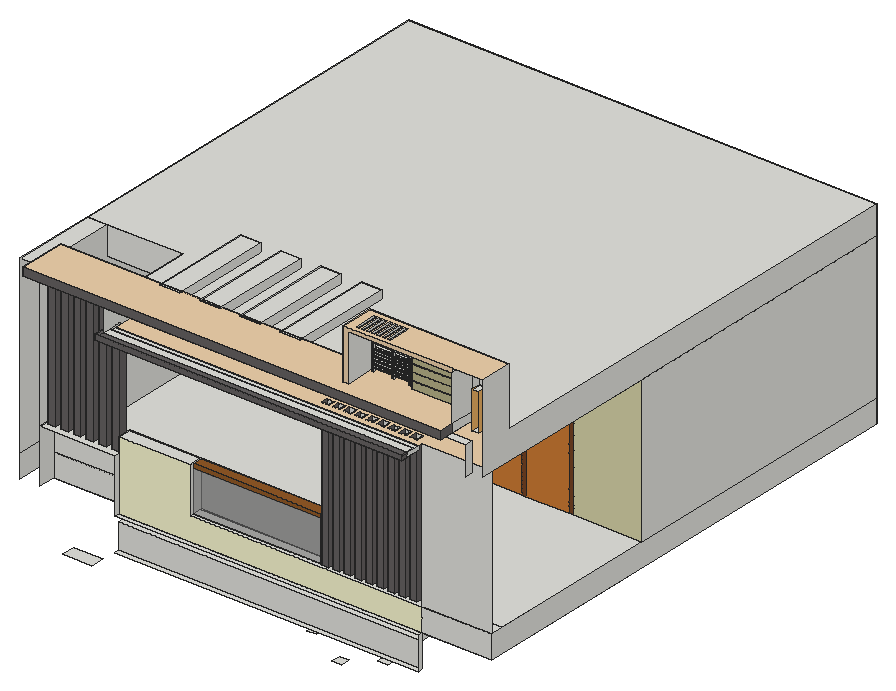
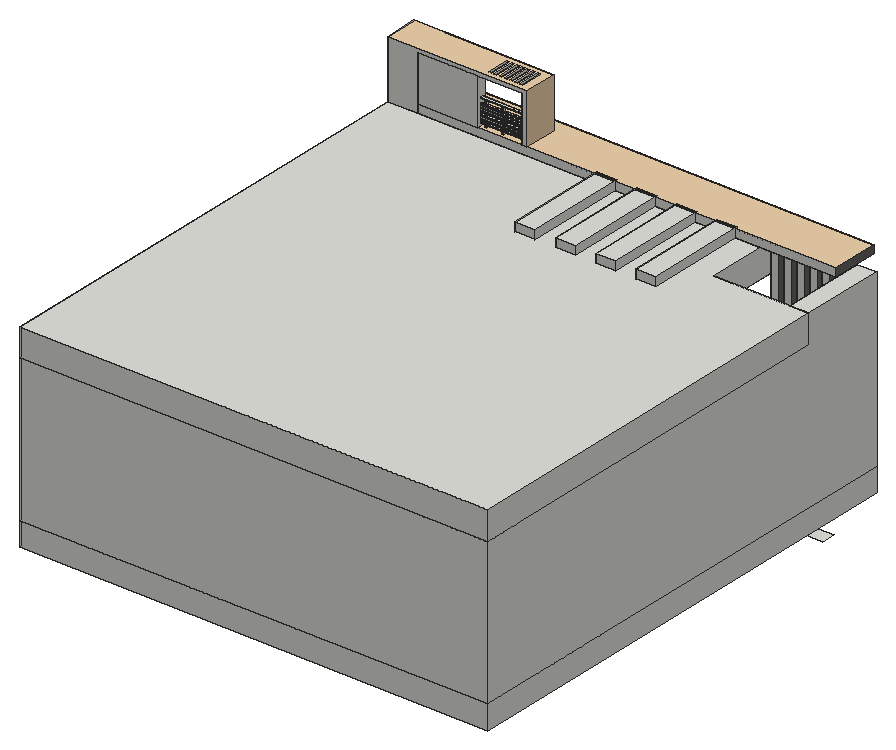
# SketchUp Ruby script. Lengths in inches.
U = 1.inch
M = Sketchup.active_model
def pt(a) = Geom::Point3d.new(a.map { |v| v * U })
def face(e, loops, mat)
  f = e.add_face(loops[0].map { |a| pt(a) })
  loops[1..].each { |l| e.add_face(l.map { |a| pt(a) }).erase! }
  f.material = f.back_material = mat if mat
  f
end
# faces: each face lists its corners as indices into pts; further lists are holes
def faces(e, pts, list, mat = nil) = list.each { |f| face(e, (f[0].is_a?(Array) ? f : [f]).map { |l| l.map { |i| pts[i] } }, mat) }
# xy, xz, yz: faces in a plane at the given z, y or x. An outline is a flat list of corners, or four numbers for a rectangle; further outlines are holes
def ring(l) = l.size == 4 ? [[l[0], l[1]], [l[2], l[1]], [l[2], l[3]], [l[0], l[3]]] : l.each_slice(2).to_a
def flat(e, list, mat, &to3) = list.each { |f| face(e, (f[0].is_a?(Array) ? f : [f]).map { |l| ring(l).map { |u, v| to3.(u, v) } }, mat) }
def xy(e, z, list, mat = nil) = flat(e, list, mat) { |x, y| [x, y, z] }
def xz(e, y, list, mat = nil) = flat(e, list, mat) { |x, z| [x, y, z] }
def yz(e, x, list, mat = nil) = flat(e, list, mat) { |y, z| [x, y, z] }
def lines(e, pts, list) = list.each { |a, b| e.add_line(pt(pts[a]), pt(pts[b])) }
# prism: a flat outline (further loops are holes) pulled along v
def prism(e, loops, v, mat = nil)
  f = face(e, loops, mat); d = Geom::Vector3d.new(v.map { |x| x * U })
  f.pushpull(f.normal.samedirection?(d) ? d.length : -d.length)
end
def box(e, o, s, mat = nil) = prism(e, [[o, [o[0] + s[0], o[1], o[2]], [o[0] + s[0], o[1] + s[1], o[2]], [o[0], o[1] + s[1], o[2]]]], [0, 0, s[2]], mat)
def at(x, y, z, deg = 0) = Geom::Transformation.translation(pt([x, y, z])) * Geom::Transformation.rotation(ORIGIN, Z_AXIS, deg.degrees)
def axes(o, x, y, z) = Geom::Transformation.new([*x, 0, *y, 0, *z, 0, *pt(o).to_a, 1])
def part(name) = M.definitions.add(name)
# library, detail: a bought-in or finely detailed component or shape, given as its bounding box
def library(name, o, s) = part(name).tap { |d| box(d.entities, o, s) }
def detail(e, o, s) = box(e.add_group.entities, o, s)
def put(e, d, t, mat = nil) = e.add_instance(d, t).tap { |i| i.material = mat if mat }
def group(e, t, mat = nil) = e.add_group.tap { |g| g.transformation = t; g.material = mat if mat }.entities
root = M.entities
M.materials.add("Generic\#1").color = [235, 176, 99]
M.materials.add("Generic\#2").color = [102, 98, 98]
M.materials.add("Generic\#3").color = [183, 179, 137]
M.materials.add("Generic\#4").color = [217, 213, 170]
M.materials.add("Generic\#6").color = [239, 209, 171]
M.materials.add("Generic\#7").color = [249, 247, 208]
M.materials.add("[Translucent Glass Gray]").color = [128, 128, 128]
M.materials["[Translucent Glass Gray]"].alpha = 0.5
M.materials.add("[Wood Bamboo]").color = [206, 124, 53]
M.materials.add("[Wood Floor Parquet]").color = [145, 89, 39]
M.materials.add("[Wood Veneer 01]").color = [119, 69, 36]
c1 = library("Group14",[-64.97,9.24,0.31],[138.52,9.93,292.57])
c2 = library("Group16",[86.37,-10.76,76.46],[21.79,14.87,35.97])
c3 = library("Group22",[48.82,-10.91,0.23],[97.72,18.57,293.12])
c4 = library("Group24",[44.03,2.01,0.26],[103.73,11,292.35])
c5 = library("Group27",[-106.21,-10.76,76.46],[21.8,14.87,35.97])
c6 = library("Group35",[-145.81,2.01,0.26],[103.73,11,292.35])
c7 = library("Group33",[-144.59,-10.91,0.23],[97.72,18.57,293.12])
c8 = part("rem (1)")
g1 = group(c8.entities,at(-145.81,-10.91,0.23))
put(g1,c1,at(145.81,10.91,-0.23))
put(g1,c2,at(145.81,10.91,-0.23))
put(g1,c3,at(145.81,10.91,-0.23))
put(g1,c4,at(145.81,10.91,-0.23))
put(g1,c5,at(145.81,10.91,-0.23))
put(g1,c6,at(145.81,10.91,-0.23))
put(g1,c7,at(145.81,10.91,-0.23))
xy(root,245.22,[[294.23,85.3125,304.04,94.5625]])
xy(root,258.96,[[42.04,67.875,71.06,81.625]])
xy(root,261.43,[[339.93,85.3125,349.75,94.5625]])
xy(root,263.68,[[269.72,85.3125,279.54,94.5625]])
xy(root,276.62,[[315.33,85.3125,325.14,94.5625]])
xy(root,277.23,[[366.08,85.3125,375.89,94.5625]])
xy(root,278.625,[[93.91,67.875,394.04,72.375]])
xy(root,286.8125,[[62.44,244.125,235.88,281.25]])
xy(root,304.1875,[[93.91,72.375,394.04,85.3125]])
xy(root,311.1875,[[93.91,67.875,394.04,72.375],[93.91,72.375,394.04,85.3125],[394.04,72.375,462.8125,85.3125]])
xy(root,311.1875,[[19.1875,85.3125,19.1875,244.125,462.8125,244.125,462.8125,94.5625,258.25,94.5625,258.25,85.3125]],"Generic\#6")
xy(root,334.375,[[[164.77,72.375,164.77,75.34,291.73,75.34,291.73,85.3125,394.04,85.3125,394.04,82.29,393.29,82.29,393.29,75.21,394.04,75.21,394.04,72.375],[291.98,75.21,299.23,82.29],[302.92,75.21,310.17,82.29],[313.86,75.21,321.11,82.29],[324.79,75.21,332.04,82.29],[335.73,75.21,342.98,82.29],[346.67,75.21,353.92,82.29],[357.92,75.21,364.86,82.29],[368.86,75.21,375.79,82.29],[379.79,75.21,386.73,82.29]],[394.04,72.375,394.04,75.21,397.67,75.21,397.67,82.29,394.04,82.29,394.04,85.3125,462.8125,85.3125,462.8125,72.375],[291.98,75.21,299.23,82.29],[302.92,75.21,310.17,82.29],[313.86,75.21,321.11,82.29],
  [324.79,75.21,332.04,82.29],[335.73,75.21,342.98,82.29],[346.67,75.21,353.92,82.29],[357.92,75.21,364.86,82.29],[368.86,75.21,375.79,82.29],
  [379.79,75.21,386.73,82.29],[393.29,75.21,394.04,82.29],[394.04,75.21,397.67,82.29],[164.77,75.34,291.73,85.3125],[19.1875,85.3125,19.1875,244.125,62.44,244.125,62.44,281.25,235.88,281.25,235.88,244.125,270.7,244.125,270.7,257.625,462.8125,257.625,462.8125,85.3125]])
xy(root,364.3125,[[[19.1875,67.875,93.91,85.3125],[21.625,74.83,29.4375,82.21],[34.25,74.83,42.0625,82.21],[46.875,74.83,54.6875,82.21],[59.5,74.83,67.3125,82.21],[72.125,74.83,79.9375,82.21],[84.75,74.83,92.5625,82.21]]])
xy(root,375.4375,[[164.77,75.34,291.73,85.3125]])
xy(root,379.375,[[93.91,72.375,164.77,85.3125]])
xy(root,379.375,[[164.77,75.34,291.73,85.3125]],"[Wood Floor Parquet]")
xy(root,454,[[62.44,244.125,235.88,281.25]])
xy(root,474.875,[[90.47,47.0625,90.47,74.83,93.91,74.83,93.91,67.875,394.04,67.875,394.04,47.0625]])
xy(root,478.375,[[93.91,60.6875,394.04,67.875],[0,151.0625,0,547.875,462.8125,547.875,462.8125,257.625,270.7,257.625,270.7,244.125,19.1875,244.125,19.1875,151.0625]])
xy(root,478.375,[[[93.91,67.875,93.91,151.0625,19.1875,151.0625,19.1875,244.125,270.7,244.125,270.7,257.625,462.8125,257.625,462.8125,72.375,394.04,72.375,394.04,67.875],[119.28,91.33,139.09,191.7],[158.97,91.33,178.78,191.7],[198.65,91.33,218.47,191.7],[238.34,91.33,258.15,191.7],[346.67,75.21,353.92,82.29],[335.73,75.21,342.98,82.29],[324.79,75.21,332.04,82.29],[313.86,75.21,321.11,82.29],[302.92,75.21,310.17,82.29],[291.98,75.21,299.23,82.29],[379.79,75.21,386.73,82.29],[368.86,75.21,375.79,82.29],[357.92,75.21,364.86,82.29]]],"Generic\#6")
xy(root,480.125,[[93.91,53.25,394.04,60.6875]])
xy(root,480.125,[[90.47,47.0625,93.91,74.83],[93.91,47.0625,394.04,53.25]],"Generic\#2")
xy(root,506.6875,[[[19.1875,47.0625,93.91,93.625],[21.625,74.83,29.4375,82.21],[34.25,74.83,42.0625,82.21],[46.875,74.83,54.6875,82.21],[59.5,74.83,67.3125,82.21],[72.125,74.83,79.9375,82.21],[84.75,74.83,92.5625,82.21]],[93.91,47.0625,432.56,53.25],[93.91,53.25,432.56,93.625],[432.56,53.25,452.8125,60.6875],[0,67.875,19.1875,151.0625],
  [93.91,93.625,462.8125,93.625,462.8125,547.875,0,547.875,0,151.0625,93.91,151.0625]])
xy(root,514.6875,[[374,85,432.56,93.625],[332.03,87.87,333.97,89.37],[351.41,87.87,353.35,89.37],[368.3,88.125,370.24,89.3125],[119.28,91.33,139.09,93.625],
  [158.97,91.33,178.78,93.625],[198.65,91.33,218.47,93.625],[238.34,91.33,258.15,93.625],[119.28,93.625,139.09,191.7],[158.97,93.625,178.78,191.7],
  [198.65,93.625,218.47,191.7],[238.34,93.625,258.15,191.7]])
xy(root,514.6875,[[[19.1875,47.0625,432.56,47.0625,432.56,85,374,85,374,93.625,330.5,93.625,330.5,60.6875,325.13,60.6875,325.13,93.625,258.15,93.625,258.15,91.33,238.34,91.33,238.34,93.625,218.47,93.625,218.47,91.33,198.65,91.33,198.65,93.625,178.78,93.625,178.78,91.33,158.97,91.33,158.97,93.625,139.09,93.625,139.09,91.33,119.28,91.33,119.28,93.625,19.1875,93.625],[351.41,87.87,353.35,89.37],[332.03,87.87,333.97,89.37],[368.3,88.125,370.24,89.3125]]],"Generic\#6")
xy(root,515.875,[[452.8125,60.6875,459.25,69.875]])
xy(root,517.37,[[330.5,87.99,374,90.49]])
xy(root,518.43,[[330.5,87.99,374,90.49]])
xy(root,519.93,[[330.5,87.99,374,90.49]])
xy(root,520.99,[[330.5,87.99,374,90.49]])
xy(root,521.79,[[374,85,432.56,85.5]])
xy(root,522.18,[[330.5,87.99,374,90.49]])
xy(root,522.29,[[374,85,432.56,85.5]])
xy(root,523.24,[[330.5,87.99,374,90.49]])
xy(root,524.74,[[330.5,87.99,374,90.49]])
xy(root,525.81,[[330.5,87.99,374,90.49]])
xy(root,527.18,[[330.5,87.99,374,90.49]])
xy(root,528.24,[[330.5,87.99,374,90.49]])
xy(root,529.37,[[330.5,87.99,374,90.49]])
xy(root,529.4,[[374,85,432.56,85.5]])
xy(root,529.9,[[374,85,432.56,85.5]])
xy(root,530.43,[[330.5,87.99,374,90.49]])
xy(root,532.06,[[330.5,87.99,374,90.49]])
xy(root,533.12,[[330.5,87.99,374,90.49]])
xy(root,534.24,[[330.5,87.99,374,90.49]])
xy(root,535.31,[[330.5,87.99,374,90.49]])
xy(root,537,[[374,85,432.56,85.5]])
xy(root,537.5,[[374,85,432.56,85.5]])
xy(root,539.4,[[330.5,87.63,374,90.07]])
xy(root,539.43,[[332.03,87.87,333.97,89.37],[351.41,87.87,353.35,89.37],[368.3,88.125,370.24,89.3125]])
xy(root,540.65,[[330.5,87.63,374,90.07]])
xy(root,544.6,[[374,85,432.56,85.5]])
xy(root,545.1,[[374,85,432.56,85.5]])
xy(root,552.21,[[374,85,432.56,85.5]])
xy(root,552.5,[[452.8125,60.6875,459.25,69.875]])
xy(root,552.71,[[374,85,432.56,85.5]])
xy(root,560.3125,[[[330.5,60.6875,374,93.625],[334.09,65.97,336.59,87.53],[339.21,65.97,341.71,87.53],[344.34,65.97,346.84,87.53],[349.46,65.97,351.96,87.53],[354.59,65.97,357.09,87.53],[359.71,65.97,362.21,87.53],[364.84,65.97,367.34,87.53]],[374,60.6875,432.56,85],[374,85,432.56,93.625]])
xy(root,564.0625,[[[325.13,60.6875,462.8125,93.625],[364.84,65.97,367.34,87.53],[359.71,65.97,362.21,87.53],[354.59,65.97,357.09,87.53],[349.46,65.97,351.96,87.53],[344.34,65.97,346.84,87.53],[339.21,65.97,341.71,87.53],[334.09,65.97,336.59,87.53]]],"Generic\#6")
xz(root,47.0625,[[90.47,474.875,394.04,480.125],[19.1875,506.6875,432.56,514.6875]],"Generic\#2")
xz(root,60.6875,[[93.91,478.375,394.04,480.125]])
xz(root,60.6875,[[325.13,514.6875,325.13,564.0625,432.56,564.0625,432.56,560.3125,330.5,560.3125,330.5,514.6875]],"Generic\#6")
xz(root,65.97,[[334.09,560.3125,336.59,564.0625],[339.21,560.3125,341.71,564.0625],[344.34,560.3125,346.84,564.0625],[349.46,560.3125,351.96,564.0625],[354.59,560.3125,357.09,564.0625],
  [359.71,560.3125,362.21,564.0625],[364.84,560.3125,367.34,564.0625]])
xz(root,67.875,[[93.91,474.875,394.04,478.375]])
xz(root,69.875,[[452.8125,515.875,459.25,552.5]],"Generic\#1")
xz(root,72.375,[[93.91,278.625,394.04,304.1875],[394.04,311.1875,462.8125,334.375],[394.04,334.375,462.8125,478.375]])
xz(root,72.375,[[93.91,311.1875,394.04,311.1875,394.04,334.375,164.77,334.375,164.77,379.375,93.91,379.375]],"Generic\#7")
xz(root,74.83,[[90.47,474.875,92.5625,480.125],[92.5625,474.875,93.91,480.125]])
xz(root,74.83,[[21.625,364.3125,29.4375,506.6875],[34.25,364.3125,42.0625,506.6875],[46.875,364.3125,54.6875,506.6875],[59.5,364.3125,67.3125,506.6875],[72.125,364.3125,79.9375,506.6875],
  [84.75,364.3125,92.5625,364.3125,92.5625,474.875,90.47,474.875,90.47,480.125,92.5625,480.125,92.5625,506.6875,84.75,506.6875]],"Generic\#2")
xz(root,75.21,[[291.98,334.375,299.23,478.375],[302.92,334.375,310.17,478.375],[313.86,334.375,321.11,478.375],[324.79,334.375,332.04,478.375],[335.73,334.375,342.98,478.375],
  [346.67,334.375,353.92,478.375],[357.92,334.375,364.86,478.375],[368.86,334.375,375.79,478.375],[379.79,334.375,386.73,478.375]],"Generic\#2")
xz(root,75.34,[[164.77,334.375,291.73,375.4375]],"[Translucent Glass Gray]")
xz(root,75.34,[[164.77,375.4375,291.73,379.375]],"[Wood Floor Parquet]")
xz(root,82.21,[[21.625,364.3125,29.4375,506.6875],[34.25,364.3125,42.0625,506.6875],[46.875,364.3125,54.6875,506.6875],[59.5,364.3125,67.3125,506.6875],[72.125,364.3125,79.9375,506.6875],
  [84.75,364.3125,92.5625,506.6875]])
xz(root,82.29,[[291.98,334.375,299.23,478.375],[302.92,334.375,310.17,478.375],[313.86,334.375,321.11,478.375],[324.79,334.375,332.04,478.375],[335.73,334.375,342.98,478.375],
  [346.67,334.375,353.92,478.375],[357.92,334.375,364.86,478.375],[368.86,334.375,375.79,478.375],[379.79,334.375,386.73,478.375]])
xz(root,85,[[374,514.6875,432.56,521.79],[374,522.29,432.56,529.4],[374,529.9,432.56,537],[374,537.5,432.56,544.6],[374,545.1,432.56,552.21],
  [374,552.71,432.56,560.3125]],"Generic\#3")
xz(root,85.3125,[[258.25,304.1875,394.04,311.1875],[19.1875,311.1875,93.91,334.375],[19.1875,334.375,93.91,364.3125],[93.91,334.375,164.77,379.375],[164.77,375.4375,291.73,379.375]])
xz(root,85.3125,[[164.77,334.375,291.73,375.4375]],"[Translucent Glass Gray]")
xz(root,85.5,[[374,521.79,432.56,522.29],[374,529.4,432.56,529.9],[374,537,432.56,537.5],[374,544.6,432.56,545.1],[374,552.21,432.56,552.71]])
xz(root,87.53,[[334.09,560.3125,336.59,564.0625],[339.21,560.3125,341.71,564.0625],[344.34,560.3125,346.84,564.0625],[349.46,560.3125,351.96,564.0625],[354.59,560.3125,357.09,564.0625],
  [359.71,560.3125,362.21,564.0625],[364.84,560.3125,367.34,564.0625]])
xz(root,87.63,[[330.5,539.4,374,540.65]])
xz(root,87.87,[[332.03,514.6875,333.97,539.43],[351.41,514.6875,353.35,539.43]])
xz(root,87.99,[[330.5,517.37,374,518.43],[330.5,519.93,374,520.99],[330.5,522.18,374,523.24],[330.5,524.74,374,525.81],[330.5,527.18,374,528.24],
  [330.5,529.37,374,530.43],[330.5,532.06,374,533.12],[330.5,534.24,374,535.31]])
xz(root,88.125,[[368.3,514.6875,370.24,539.43]])
xz(root,89.3125,[[368.3,514.6875,370.24,539.43]])
xz(root,89.37,[[332.03,514.6875,333.97,539.43],[351.41,514.6875,353.35,539.43]])
xz(root,90.07,[[330.5,539.4,374,540.65]])
xz(root,90.49,[[330.5,517.37,374,518.43],[330.5,519.93,374,520.99],[330.5,522.18,374,523.24],[330.5,524.74,374,525.81],[330.5,527.18,374,528.24],
  [330.5,529.37,374,530.43],[330.5,532.06,374,533.12],[330.5,534.24,374,535.31]])
xz(root,91.33,[[119.28,478.375,139.09,514.6875],[158.97,478.375,178.78,514.6875],[198.65,478.375,218.47,514.6875],[238.34,478.375,258.15,514.6875]])
xz(root,93.625,[[19.1875,506.6875,432.56,514.6875],[432.56,506.6875,462.8125,506.6875,462.8125,564.0625,325.13,564.0625,325.13,514.6875,330.5,514.6875,330.5,560.3125,432.56,560.3125],[374,514.6875,432.56,560.3125]])
xz(root,151.0625,[[0,478.375,19.1875,506.6875],[19.1875,478.375,93.91,506.6875]])
xz(root,191.7,[[119.28,478.375,139.09,514.6875],[158.97,478.375,178.78,514.6875],[198.65,478.375,218.47,514.6875],[238.34,478.375,258.15,514.6875]])
xz(root,244.125,[[19.1875,334.375,62.44,334.375,62.44,454,235.88,454,235.88,334.375,270.7,334.375,270.7,478.375,19.1875,478.375]],"Generic\#4")
xz(root,257.625,[[270.7,334.375,297.63,334.375,297.63,456.8125,395.32,456.8125,395.32,334.375,462.8125,334.375,462.8125,478.375,270.7,478.375]],"Generic\#4")
xz(root,257.625,[[302.3125,334.375,344.47,452.13],[348.47,334.375,390.63,452.13]],"[Wood Bamboo]")
xz(root,257.625,[[297.63,334.375,302.3125,334.375,302.3125,452.13,390.63,452.13,390.63,334.375,395.32,334.375,395.32,456.8125,297.63,456.8125],[344.47,334.375,348.47,452.13]],"[Wood Veneer 01]")
xz(root,281.25,[[62.44,334.375,235.88,454]])
xz(root,547.875,[[0,311.1875,462.8125,334.375],[0,334.375,462.8125,478.375],[0,478.375,462.8125,506.6875]])
yz(root,0,[[67.875,311.1875,547.875,334.375],[67.875,334.375,67.875,506.6875,151.0625,506.6875,151.0625,478.375,547.875,478.375,547.875,334.375],[151.0625,478.375,547.875,506.6875]])
yz(root,19.1875,[[67.875,311.1875,85.3125,364.3125],[85.3125,334.375,244.125,334.375,244.125,478.375,151.0625,478.375,151.0625,506.6875,67.875,506.6875,67.875,364.3125,85.3125,364.3125]])
yz(root,19.1875,[[47.0625,506.6875,93.625,514.6875]],"Generic\#2")
yz(root,21.625,[[74.83,364.3125,82.21,506.6875]])
yz(root,29.4375,[[74.83,364.3125,82.21,506.6875]],"Generic\#2")
yz(root,34.25,[[74.83,364.3125,82.21,506.6875]],"Generic\#2")
yz(root,42.0625,[[74.83,364.3125,82.21,506.6875]],"Generic\#2")
yz(root,46.875,[[74.83,364.3125,82.21,506.6875]],"Generic\#2")
yz(root,54.6875,[[74.83,364.3125,82.21,506.6875]],"Generic\#2")
yz(root,59.5,[[74.83,364.3125,82.21,506.6875]],"Generic\#2")
yz(root,62.44,[[244.125,334.375,281.25,454]])
yz(root,67.3125,[[74.83,364.3125,82.21,506.6875]],"Generic\#2")
yz(root,72.125,[[74.83,364.3125,82.21,506.6875]],"Generic\#2")
yz(root,79.9375,[[74.83,364.3125,82.21,506.6875]],"Generic\#2")
yz(root,84.75,[[74.83,364.3125,82.21,506.6875]],"Generic\#2")
yz(root,90.47,[[47.0625,474.875,74.83,480.125]],"Generic\#2")
yz(root,92.5625,[[74.83,364.3125,82.21,506.6875]],"Generic\#2")
yz(root,93.91,[[67.875,311.1875,72.375,364.3125],[72.375,311.1875,85.3125,364.3125],[72.375,364.3125,85.3125,379.375],[67.875,474.875,74.83,478.375],[74.83,478.375,74.83,480.125,53.25,480.125,53.25,506.6875,151.0625,506.6875,151.0625,478.375],
  [60.6875,478.375,74.83,480.125]])
yz(root,119.28,[[91.33,478.375,191.7,514.6875]])
yz(root,139.09,[[91.33,478.375,191.7,514.6875]])
yz(root,158.97,[[91.33,478.375,191.7,514.6875]])
yz(root,164.77,[[72.375,334.375,75.34,379.375],[75.34,334.375,85.3125,375.4375],[75.34,375.4375,85.3125,379.375]])
yz(root,178.78,[[91.33,478.375,191.7,514.6875]])
yz(root,198.65,[[91.33,478.375,191.7,514.6875]])
yz(root,218.47,[[91.33,478.375,191.7,514.6875]])
yz(root,235.88,[[244.125,334.375,281.25,454]])
yz(root,238.34,[[91.33,478.375,191.7,514.6875]])
yz(root,258.15,[[91.33,478.375,191.7,514.6875]])
yz(root,270.7,[[244.125,334.375,257.625,478.375]])
yz(root,291.73,[[75.34,334.375,85.3125,375.4375],[75.34,375.4375,85.3125,379.375]])
yz(root,291.98,[[75.21,334.375,82.29,478.375]],"Generic\#2")
yz(root,299.23,[[75.21,334.375,82.29,478.375]],"Generic\#2")
yz(root,302.92,[[75.21,334.375,82.29,478.375]],"Generic\#2")
yz(root,310.17,[[75.21,334.375,82.29,478.375]],"Generic\#2")
yz(root,313.86,[[75.21,334.375,82.29,478.375]],"Generic\#2")
yz(root,321.11,[[75.21,334.375,82.29,478.375]],"Generic\#2")
yz(root,324.79,[[75.21,334.375,82.29,478.375]],"Generic\#2")
yz(root,325.13,[[60.6875,514.6875,93.625,564.0625]],"Generic\#6")
yz(root,330.5,[[[60.6875,514.6875,93.625,560.3125],[87.63,539.4,90.07,540.65],[87.99,534.24,90.49,535.31],[87.99,532.06,90.49,533.12],[87.99,529.37,90.49,530.43],[87.99,527.18,90.49,528.24],[87.99,524.74,90.49,525.81],[87.99,522.18,90.49,523.24],[87.99,519.93,90.49,520.99],[87.99,517.37,90.49,518.43]]])
yz(root,332.03,[[87.87,514.6875,89.37,539.43]])
yz(root,332.04,[[75.21,334.375,82.29,478.375]],"Generic\#2")
yz(root,333.97,[[87.87,514.6875,89.37,539.43]])
yz(root,334.09,[[65.97,560.3125,87.53,564.0625]])
yz(root,335.73,[[75.21,334.375,82.29,478.375]],"Generic\#2")
yz(root,336.59,[[65.97,560.3125,87.53,564.0625]])
yz(root,339.21,[[65.97,560.3125,87.53,564.0625]])
yz(root,341.71,[[65.97,560.3125,87.53,564.0625]])
yz(root,342.98,[[75.21,334.375,82.29,478.375]],"Generic\#2")
yz(root,344.34,[[65.97,560.3125,87.53,564.0625]])
yz(root,346.67,[[75.21,334.375,82.29,478.375]],"Generic\#2")
yz(root,346.84,[[65.97,560.3125,87.53,564.0625]])
yz(root,349.46,[[65.97,560.3125,87.53,564.0625]])
yz(root,351.41,[[87.87,514.6875,89.37,539.43]])
yz(root,351.96,[[65.97,560.3125,87.53,564.0625]])
yz(root,353.35,[[87.87,514.6875,89.37,539.43]])
yz(root,353.92,[[75.21,334.375,82.29,478.375]],"Generic\#2")
yz(root,354.59,[[65.97,560.3125,87.53,564.0625]])
yz(root,357.09,[[65.97,560.3125,87.53,564.0625]])
yz(root,357.92,[[75.21,334.375,82.29,478.375]],"Generic\#2")
yz(root,359.71,[[65.97,560.3125,87.53,564.0625]])
yz(root,362.21,[[65.97,560.3125,87.53,564.0625]])
yz(root,364.84,[[65.97,560.3125,87.53,564.0625]])
yz(root,364.86,[[75.21,334.375,82.29,478.375]],"Generic\#2")
yz(root,367.34,[[65.97,560.3125,87.53,564.0625]])
yz(root,368.3,[[88.125,514.6875,89.3125,539.43]])
yz(root,368.86,[[75.21,334.375,82.29,478.375]],"Generic\#2")
yz(root,370.24,[[88.125,514.6875,89.3125,539.43]])
yz(root,374,[[[85,514.6875,85,521.79,85.5,521.79,85.5,522.29,85,522.29,85,529.4,85.5,529.4,85.5,529.9,85,529.9,85,537,85.5,537,85.5,537.5,85,537.5,85,544.6,85.5,544.6,85.5,545.1,85,545.1,85,552.21,85.5,552.21,85.5,552.71,85,552.71,85,560.3125,93.625,560.3125,93.625,514.6875],[87.63,539.4,90.07,540.65],[87.99,534.24,90.49,535.31],[87.99,532.06,90.49,533.12],[87.99,529.37,90.49,530.43],[87.99,527.18,90.49,528.24],[87.99,524.74,90.49,525.81],[87.99,522.18,90.49,523.24],[87.99,519.93,90.49,520.99],[87.99,517.37,90.49,518.43]],[87.99,517.37,90.49,518.43],[87.99,519.93,90.49,520.99],[87.99,522.18,90.49,523.24],[87.99,524.74,90.49,525.81],
  [87.99,527.18,90.49,528.24],[87.99,529.37,90.49,530.43],[87.99,532.06,90.49,533.12],[87.99,534.24,90.49,535.31]])
yz(root,375.79,[[75.21,334.375,82.29,478.375]],"Generic\#2")
yz(root,379.79,[[75.21,334.375,82.29,478.375]],"Generic\#2")
yz(root,386.73,[[75.21,334.375,82.29,478.375]],"Generic\#2")
yz(root,394.04,[[67.875,278.625,72.375,311.1875],[72.375,304.1875,85.3125,311.1875],[53.25,474.875,67.875,478.375],[53.25,478.375,60.6875,480.125]])
yz(root,394.04,[[47.0625,474.875,53.25,478.375],[47.0625,478.375,53.25,480.125]],"Generic\#2")
yz(root,432.56,[[60.6875,506.6875,93.625,514.6875],[60.6875,514.6875,85,514.6875,85,521.79,85.5,521.79,85.5,522.29,85,522.29,85,529.4,85.5,529.4,85.5,529.9,85,529.9,85,537,85.5,537,85.5,537.5,85,537.5,85,544.6,85.5,544.6,85.5,545.1,85,545.1,85,552.21,85.5,552.21,85.5,552.71,85,552.71,85,560.3125,60.6875,560.3125],[85,514.6875,93.625,514.6875,93.625,560.3125,85,560.3125,85,552.71,85.5,552.71,85.5,552.21,85,552.21,85,545.1,85.5,545.1,85.5,544.6,85,544.6,85,537.5,85.5,537.5,85.5,537,85,537,85,529.9,85.5,529.9,85.5,529.4,85,529.4,85,522.29,85.5,522.29,85.5,521.79,85,521.79]])
yz(root,432.56,[[47.0625,506.6875,60.6875,514.6875]],"Generic\#2")
yz(root,452.8125,[[53.25,478.375,60.6875,506.6875]])
yz(root,452.8125,[[60.6875,515.875,69.875,552.5]],"Generic\#1")
yz(root,459.25,[[60.6875,515.875,69.875,552.5]],"Generic\#1")
yz(root,462.8125,[[72.375,311.1875,547.875,334.375],[257.625,334.375,547.875,478.375],[60.6875,478.375,547.875,478.375,547.875,506.6875,93.625,506.6875,93.625,564.0625,60.6875,564.0625]])
p = [[238.01,255.51,305.4],[64.58,255.51,305.4],[374,89.09,517.86],[330.5,89.09,517.86],[374,89.09,520.3],[330.5,89.09,520.3],
  [374,89.09,522.74],[330.5,89.09,522.74],[374,89.09,525.18],[330.5,89.09,525.18],[374,89.09,527.61],[330.5,89.09,527.61],
  [374,89.09,530.05],[330.5,89.09,530.05],[374,89.09,532.49],[330.5,89.09,532.49],[374,89.09,534.93],[330.5,89.09,534.93]]
lines(root,p,[[0,1],[2,3],[4,5],[6,7],[8,9],[10,11],[12,13],[14,15],[16,17]])
put(root,c8,axes([151.59,269.39,304.39],[0.59078,0,0],[0,0.51,0],[0,0,0.51]))
g2 = group(root,at(62.44,244.125,334.375),"Generic\#6")
xz(g2,0,[[40.6,4.85,168.59,114.77],[7.87,7.87,27.88,111.75]],"[Translucent Glass Gray]")
xz(g2,0,[[[0,0,35.75,119.625],[7.87,7.87,27.88,111.75]],[[35.75,0,173.4375,119.625],[40.6,4.85,168.59,114.77]]],"[Wood Veneer 01]")
